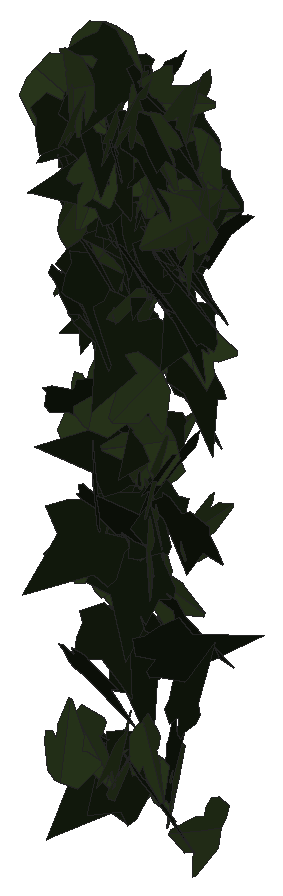
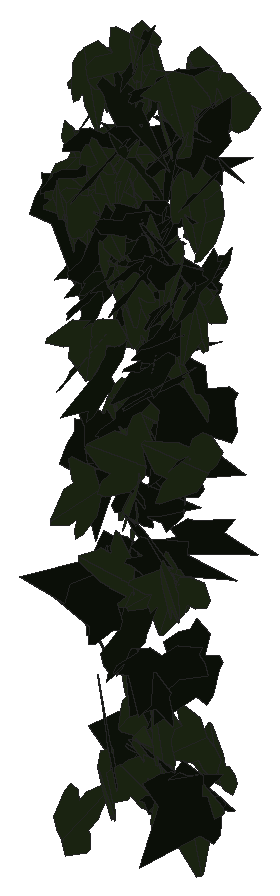
# SketchUp Ruby script. Lengths in inches.
U = 1.inch
M = Sketchup.active_model
def pt(a) = Geom::Point3d.new(a.map { |v| v * U })
def face(e, loops, mat)
  f = e.add_face(loops[0].map { |a| pt(a) })
  loops[1..].each { |l| e.add_face(l.map { |a| pt(a) }).erase! }
  f.material = f.back_material = mat if mat
  f
end
# faces: each face lists its corners as indices into pts; further lists are holes
def faces(e, pts, list, mat = nil) = list.each { |f| face(e, (f[0].is_a?(Array) ? f : [f]).map { |l| l.map { |i| pts[i] } }, mat) }
# xy, xz, yz: faces in a plane at the given z, y or x. An outline is a flat list of corners, or four numbers for a rectangle; further outlines are holes
def ring(l) = l.size == 4 ? [[l[0], l[1]], [l[2], l[1]], [l[2], l[3]], [l[0], l[3]]] : l.each_slice(2).to_a
def flat(e, list, mat, &to3) = list.each { |f| face(e, (f[0].is_a?(Array) ? f : [f]).map { |l| ring(l).map { |u, v| to3.(u, v) } }, mat) }
def xy(e, z, list, mat = nil) = flat(e, list, mat) { |x, y| [x, y, z] }
def xz(e, y, list, mat = nil) = flat(e, list, mat) { |x, z| [x, y, z] }
def yz(e, x, list, mat = nil) = flat(e, list, mat) { |y, z| [x, y, z] }
def lines(e, pts, list) = list.each { |a, b| e.add_line(pt(pts[a]), pt(pts[b])) }
# prism: a flat outline (further loops are holes) pulled along v
def prism(e, loops, v, mat = nil)
  f = face(e, loops, mat); d = Geom::Vector3d.new(v.map { |x| x * U })
  f.pushpull(f.normal.samedirection?(d) ? d.length : -d.length)
end
def box(e, o, s, mat = nil) = prism(e, [[o, [o[0] + s[0], o[1], o[2]], [o[0] + s[0], o[1] + s[1], o[2]], [o[0], o[1] + s[1], o[2]]]], [0, 0, s[2]], mat)
def at(x, y, z, deg = 0) = Geom::Transformation.translation(pt([x, y, z])) * Geom::Transformation.rotation(ORIGIN, Z_AXIS, deg.degrees)
def axes(o, x, y, z) = Geom::Transformation.new([*x, 0, *y, 0, *z, 0, *pt(o).to_a, 1])
def part(name) = M.definitions.add(name)
# library, detail: a bought-in or finely detailed component or shape, given as its bounding box
def library(name, o, s) = part(name).tap { |d| box(d.entities, o, s) }
def detail(e, o, s) = box(e.add_group.entities, o, s)
def put(e, d, t, mat = nil) = e.add_instance(d, t).tap { |i| i.material = mat if mat }
def group(e, t, mat = nil) = e.add_group.tap { |g| g.transformation = t; g.material = mat if mat }.entities
root = M.entities
M.materials.add("efeu1").color = [18, 25, 13]
M.materials.add("efeu2").color = [43, 57, 29]
c1 = part("ivyleaf_10")
p = [[0,0.5,-0.03],[-0.0625,2.02,-0.43],[-0.19,2.01,-0.46],[-0.54,1.05,-0.29],[-0.52,0.625,-0.18],[-0.83,0.76,-0.28],
  [-1.16,0.64,-0.33],[-1.15,0.33,-0.24],[-0.77,-0.39,0.02],[-0.3,-0.51,0.16],[0.04,-0.48,0.23],[-0.02,2.01,-0.4375],
  [-0.06,2.01,-0.43],[0.04,-0.49,0.23],[0.67,-0.49,0.14],[1.38,0.36,-0.2],[1.375,0.51,-0.24],[0.81,0.65,-0.19],
  [0.62,0.59,-0.15],[0.6,1.09,-0.28],[0.5,1.23,-0.31]]
faces(c1.entities,p,[[0,1,2,3,4,5,6,7,8,9,10],[11,12,0,13,14,15,16,17,18,19,20]],"efeu2")
c2 = part("ivyleaf_9")
p = [[1.54,2.16,1.25],[1.36,2.04,1.19],[-0.21,0.99,0.68],[-0.71,1.11,0.82],[-0.85,0.86,0.67],[-0.8,0.17,0.21],
  [-0.9,-0.01,0.1],[-0.67,-0.16,-0.02],[-0.08,-0.08,-0.05],[-0.03,-0.6,-0.4],[0.65,-0.88,-0.66],[0.83,-0.6,-0.49],
  [1.29,-0.42,-0.43],[1.8125,-0.07,-0.26],[1.21,0.44,0.15]]
faces(c2.entities,p,[[0,1,2,3,4,5,6,7,8,9,10,11,12,13,14]],"efeu1")
put(root,c1,axes([545.26,133.13,204.74],[-0.73909,0.23851,-0.3664],[0.3295,-0.16911,-0.77474],[-0.28734,-0.8074,0.05403]))
put(root,c1,axes([544.99,133.21,205.54],[0.29961,-0.81599,-0.04519],[-0.01203,0.04372,-0.86925],[0.81715,0.29983,0.00377]))
put(root,c2,axes([543.49,133.3125,192.88],[0.70059,0.05502,-0.37636],[0.37495,0.0327,0.70274],[0.06394,-0.79461,0.00286]))
put(root,c2,axes([544.64,133.57,199.95],[0.16686,-0.43211,0.71695],[0.45253,-0.56846,-0.44793],[0.70424,0.46767,0.11797]))
put(root,c2,axes([544.91,133.45,185.375],[0.48118,-0.55843,0.45126],[0.31159,-0.32699,-0.73689],[0.64683,0.57293,0.01927]))
put(root,c1,axes([545.18,133.15,197.3],[0.75679,-0.1709,-0.51183],[-0.48636,0.16585,-0.77451],[0.23373,0.89844,0.04562]))
put(root,c2,axes([543.22,133.73,191.91],[-0.63725,-0.47299,0.3462],[-0.25265,-0.2398,-0.79267],[0.52891,-0.68443,0.03847]))
put(root,c2,axes([542.52,133.125,199.37],[0.64655,-0.50733,-0.14909],[-0.09453,0.1208,-0.82105],[0.52027,0.65243,0.03609]))
put(root,c1,axes([543.21,132.95,205.28],[0.4039,-0.29481,-0.75471],[-0.61213,0.44146,-0.50005],[0.53084,0.73337,-0.00238]))
put(root,c2,axes([542.51,133.1,204.4375],[0.22259,-0.6267,-0.48664],[-0.07771,0.48577,-0.66114],[0.78964,0.22447,0.07211]))
put(root,c2,axes([544.32,133.73,198.39],[-0.53061,-0.67232,0.03547],[-0.01566,-0.03283,-0.85644],[0.67308,-0.53078,0.00804]))
put(root,c2,axes([545.4,133.03,205.05],[0.58579,-0.41864,-0.46192],[-0.30593,0.35923,-0.71354],[0.54317,0.65382,0.09628]))
put(root,c1,axes([543.05,133.1,204.71],[0.21401,-0.77882,-0.38187],[-0.10431,0.36736,-0.80768],[0.86111,0.23806,-0.00294]))
put(root,c1,axes([543.54,133.51,202.82],[0.44771,0.61092,-0.37702],[-0.20562,-0.31658,-0.75716],[-0.68781,0.4923,-0.01905]))
put(root,c2,axes([543.67,133.93,202.38],[-0.44901,-0.2473,0.7023],[-0.53972,-0.45686,-0.50594],[0.51292,-0.69722,0.08242]))
put(root,c2,axes([543.7,132.96,193.08],[0.0254,-0.26099,0.79603],[-0.07396,0.79259,0.26222],[-0.83446,-0.0782,0.00099]))
put(root,c1,axes([542.08,133.04,204.95],[0.42676,0.39564,0.752],[0.5705,0.49024,-0.58168],[-0.62973,0.71225,-0.01735]))
put(root,c1,axes([542.36,133.32,185.08],[0.83855,-0.13043,0.06033],[-0.05943,0.01043,0.84864],[-0.13085,-0.84066,0.00117]))
put(root,c1,axes([545.11,133.79,194.97],[0.46052,-0.62325,0.36788],[0.21487,-0.29863,-0.77492],[0.69109,0.50817,-0.00421]))
put(root,c1,axes([544.62,133.9,192.15],[-0.2474,0.36892,-0.73202],[0.31239,-0.6645,-0.44047],[-0.75788,-0.39433,0.0574]))
put(root,c1,axes([546.15,133.71,202.07],[-0.45461,-0.26856,0.6914],[-0.59262,-0.35615,-0.528],[0.44605,-0.7469,0.00316]))
put(root,c1,axes([543.24,133.42,195.62],[0.89242,-0.0937,-0.04669],[0.04644,-0.00485,0.89732],[-0.09383,-0.89363,0.00002]))
put(root,c1,axes([542.63,133.59,186.08],[0.49171,-0.02456,0.68501],[0.68531,0.03446,-0.49069],[-0.01369,0.84252,0.04004]))
put(root,c2,axes([542.83,133.29,188.33],[0.83916,-0.04245,-0.15527],[-0.15511,0.00708,-0.84024],[0.04303,0.85338,-0.00075]))
put(root,c2,axes([542.99,133.92,199.3],[0.14803,-0.85599,0.04688],[0.00548,-0.04663,-0.86869],[0.85725,0.14811,-0.00254]))
put(root,c1,axes([544.72,133.27,205.25],[0.13251,-0.7053,-0.48967],[-0.04739,0.4887,-0.71674],[0.85731,0.13603,0.03606]))
put(root,c2,axes([542.89,134.07,204.01],[0.07415,-0.85093,0.24891],[0.08796,-0.24149,-0.85175],[0.88221,0.0956,0.06401]))
put(root,c1,axes([543.62,133.83,204.17],[0.44375,-0.69965,0.2326],[0.12937,-0.19337,-0.82849],[0.72586,0.4622,0.00547]))
put(root,c2,axes([543.74,133.8,194.39],[-0.35876,0.03215,-0.71065],[-0.46719,-0.61085,0.20822],[-0.53645,0.51048,0.29391]))
put(root,c2,axes([546.09,133.41,193.57],[0.61284,0.18657,-0.5871],[-0.55834,-0.18167,-0.64056],[-0.26028,0.82901,-0.00825]))
put(root,c1,axes([544.5,133.85,186.39],[0.5136,-0.20518,0.64934],[0.63378,-0.15352,-0.5498],[0.24913,0.81355,0.06002]))
put(root,c1,axes([545.0625,133.74,195.23],[0.29192,0.05176,-0.75248],[-0.75328,-0.02097,-0.29367],[-0.0383,0.80684,0.04064]))
put(root,c1,axes([542.68,133.07,201.18],[0.15612,-0.25999,0.8628],[-0.41146,0.75847,0.303],[-0.8017,-0.43991,0.01251]))
put(root,c2,axes([542.8,133.26,196.11],[0.76405,0.57437,-0.04188],[-0.03362,-0.02498,-0.95586],[-0.57491,0.76479,0.00023]))
put(root,c2,axes([544.22,133.97,191.26],[-0.62604,-0.38377,-0.42316],[0.35019,0.23817,-0.7341],[0.45134,-0.71712,-0.01735]))
put(root,c2,axes([545.48,133.29,189.31],[0.38674,0.04129,0.82396],[0.7785,0.28292,-0.37958],[-0.27305,0.86513,0.08481]))
put(root,c2,axes([543.23,133.98,204.14],[-0.82081,0.04865,0.0752],[-0.07716,-0.03199,-0.82144],[-0.04548,-0.82362,0.03634]))
put(root,c2,axes([545.89,133.59,187.72],[-0.3688,0.59982,0.41627],[0.17633,-0.37938,0.70289],[0.7085,0.40664,0.04175]))
put(root,c2,axes([544.6,133.86,205.49],[0.56903,-0.60883,-0.02337],[-0.00629,0.0261,-0.83324],[0.60925,0.56891,0.01323]))
put(root,c2,axes([543.14,134.33,184.7],[-0.56529,-0.54835,0.28499],[-0.19588,-0.20733,-0.78746],[0.58612,-0.59815,0.01169]))
put(root,c2,axes([544.2,134.11,203.75],[0.38536,-0.74928,0.17655],[0.09013,-0.15217,-0.84251],[0.76451,0.39562,0.01033]))
put(root,c2,axes([543.06,133.83,203.65],[-0.36215,-0.3754,-0.68405],[0.4695,0.49752,-0.5216],[0.62324,-0.59293,-0.00456]))
put(root,c1,axes([543.8125,133.78,186.1],[0.2999,-0.88965,-0.21557],[-0.0663,0.20514,-0.93883],[0.91299,0.30713,0.00263]))
put(root,c2,axes([542.88,134.4,199.32],[-0.16641,-0.83006,0.24522],[-0.0451,-0.24106,-0.84657],[0.86435,-0.17239,0.00304]))
put(root,c1,axes([542.77,133.18,204.2],[0.03536,-0.15347,-0.87719],[-0.02897,0.87721,-0.15465],[0.89004,0.03465,0.02981]))
put(root,c2,axes([541.95,134.3,203.98],[-0.03631,-0.36872,0.77727],[0.45731,-0.66722,-0.29515],[0.72868,0.40036,0.22396]))
put(root,c2,axes([544.22,134,185.27],[-0.89094,0.21213,0.14268],[-0.13911,0.03176,-0.91585],[-0.21449,-0.90174,0.00131]))
put(root,c2,axes([543.39,134.47,205.5],[-0.43202,-0.68704,0.20937],[0.01096,-0.25061,-0.79974],[0.71815,-0.40948,0.13815]))
put(root,c1,axes([544,133.45,185.14],[0.37935,-0.47502,0.61192],[-0.20709,0.59437,0.58977],[-0.74646,-0.4063,0.14736]))
put(root,c1,axes([546.04,133.62,201.35],[0.51913,-0.39042,-0.56565],[-0.29599,0.51277,-0.62557],[0.62031,0.57142,0.17488]))
put(root,c1,axes([544.08,134.28,198.7],[0.05027,-0.79253,0.32776],[0.01841,-0.32725,-0.79412],[0.85743,0.05349,-0.00216]))
put(root,c2,axes([544.97,134,192.64],[-0.36227,0.10427,0.71846],[-0.69085,0.19728,-0.37698],[-0.22314,-0.78007,0.00069]))
put(root,c2,axes([545.38,134.04,194.77],[-0.38805,0.70584,-0.3151],[0.15047,-0.27685,-0.80548],[-0.7582,-0.4162,0.00142]))
put(root,c1,axes([544.87,133.5,205.08],[0.09087,0.04144,0.86809],[0.34663,0.79867,-0.07441],[-0.79696,0.3521,0.06661]))
put(root,c2,axes([542.4,134.1,202.4],[0.39181,-0.69102,-0.30617],[-0.12159,0.28275,-0.79375],[0.74597,0.40904,0.03143]))
put(root,c2,axes([544.45,134.73,195.43],[-0.22738,-0.66168,0.42526],[-0.14163,-0.40099,-0.69966],[0.7737,-0.26786,-0.0031]))
put(root,c2,axes([545.1,134.5625,198.66],[0.29652,-0.64631,0.47825],[0.24114,-0.41478,-0.71005],[0.767,0.38027,0.03835]))
put(root,c1,axes([544.37,134.24,193.26],[-0.42336,0.58806,-0.38068],[0.23513,-0.29971,-0.72447],[-0.65988,-0.48408,-0.01391]))
put(root,c2,axes([543.36,133.77,203.89],[0.34514,0.03695,-0.78352],[-0.76108,0.2229,-0.32475],[0.1898,0.82664,0.12259]))
put(root,c2,axes([545.3,134.87,198.83],[-0.16361,-0.68831,0.45102],[-0.0279,-0.45495,-0.70442],[0.82245,-0.15236,0.06582]))
put(root,c1,axes([542.78,134.24,199.53],[-0.65153,0.00173,0.47916],[-0.47436,-0.11656,-0.64458],[0.06768,-0.80031,0.09491]))
put(root,c1,axes([542.7,134.24,184.58],[-0.85532,-0.0793,0.43208],[-0.42979,-0.04455,-0.85897],[0.09086,-0.95722,0.00418]))
put(root,c1,axes([542.42,134.43,202.77],[0.02978,-0.835,-0.01775],[-0.0081,0.01748,-0.83549],[0.83515,0.02995,-0.00747]))
put(root,c2,axes([543.22,134.85,197.48],[-0.11185,0.03204,0.78495],[-0.01594,-0.7928,0.03009],[0.78544,-0.01152,0.11239]))
put(root,c1,axes([545.63,134.48,205.3],[0.03978,-0.84546,-0.01075],[0.01246,0.01134,-0.8463],[0.84544,0.03961,0.01298]))
put(root,c1,axes([544.48,134.47,190.57],[0.01134,-0.05015,0.84447],[0.84544,0.03013,-0.00957],[-0.02951,0.84401,0.05051]))
put(root,c2,axes([541.82,134.72,200.05],[0.39018,-0.6508,0.27175],[0.1751,-0.21145,-0.7578],[0.68318,0.42589,0.03902]))
put(root,c1,axes([542.29,134.18,199.47],[-0.11698,-0.72728,-0.411],[0.04774,0.40851,-0.73646],[0.83401,-0.12539,-0.01549]))
put(root,c2,axes([544.7,134.57,189.84],[0.57457,-0.35446,0.51902],[0.42482,-0.29923,-0.67465],[0.4632,0.71413,-0.02507]))
put(root,c1,axes([544.21,134.5,202.71],[-0.70565,-0.39815,0.0833],[-0.01467,-0.14177,-0.80193],[0.40651,-0.69626,0.11566]))
put(root,c2,axes([544.74,134.5625,200.58],[-0.60341,0.11226,0.59349],[-0.58622,0.09324,-0.61366],[-0.1455,-0.84121,0.01119]))
put(root,c2,axes([543.63,134.61,188.15],[-0.41231,-0.12852,-0.71929],[0.69162,0.19778,-0.43178],[0.2357,-0.80514,0.00875]))
put(root,c1,axes([544.08,134.59,185.01],[0.60264,0.19496,-0.51579],[-0.50873,-0.09817,-0.6315],[-0.21272,0.78713,0.04899]))
put(root,c2,axes([542.99,134.92,201.16],[0.18704,-0.76002,0.2687],[0.03922,-0.26693,-0.78232],[0.80517,0.18956,-0.02431]))
put(root,c1,axes([543.01,134.25,190.92],[0.44414,0.17752,0.63939],[0.5357,0.35813,-0.47155],[-0.39161,0.69124,0.08011]))
put(root,c2,axes([545.35,134.83,197.03],[0.26692,-0.78194,0.14398],[0.05403,-0.13369,-0.82621],[0.79325,0.27222,0.00783]))
put(root,c1,axes([545.93,134.32,202.47],[0.63157,-0.41535,-0.36935],[-0.18522,0.36983,-0.73262],[0.52405,0.63128,0.18618]))
put(root,c1,axes([542.5,133.95,194.29],[0.33461,0.38881,-0.75083],[0.50467,0.55604,0.51284],[0.6784,-0.60542,-0.01118]))
put(root,c2,axes([543.37,134.92,191.82],[-0.69139,-0.18242,0.44208],[-0.41893,-0.14383,-0.71453],[0.23068,-0.80794,0.02739]))
put(root,c2,axes([543.09,134.53,197.82],[-0.35852,-0.71787,0.36931],[0.22594,0.29872,0.79999],[-0.77504,0.41916,0.06238]))
put(root,c1,axes([545.66,135,202.08],[-0.24937,-0.52013,0.57878],[-0.0395,-0.59853,-0.55489],[0.77715,-0.19733,0.15751]))
put(root,c2,axes([544.54,134.79,185.04],[-0.06285,0.3839,0.76711],[0.12279,-0.75722,0.38901],[0.84898,0.13794,0.00052]))
put(root,c2,axes([544.53,134.34,203.32],[-0.50132,0.59775,0.24254],[-0.21572,0.13415,-0.77648],[-0.60794,-0.54051,0.07551]))
put(root,c1,axes([542.76,134.45,190.96],[0.63349,0.48756,0.24177],[0.1917,0.14733,-0.79939],[-0.50933,0.66186,-0.00016]))
put(root,c2,axes([544.52,134.54,200.06],[0.69505,-0.40928,0.03289],[0.03139,-0.01152,-0.80658],[0.4094,0.69573,0.006]))
put(root,c1,axes([544.55,134.96,200.51],[0.21843,-0.67264,0.43846],[0.14946,-0.41239,-0.70711],[0.7889,0.26437,0.01256]))
put(root,c2,axes([543.74,135.11,189.17],[0.69611,-0.36773,-0.47611],[0.41872,-0.22665,0.78726],[-0.43195,-0.81233,-0.00412]))
put(root,c2,axes([544.84,134.6,200.4],[0.66468,-0.45827,0.05261],[0.05435,-0.01384,-0.80712],[0.45807,0.66661,0.01942]))
put(root,c1,axes([542.8,134.57,205.73],[0.81786,0.08517,-0.1711],[-0.18267,0.12717,-0.80986],[-0.05622,0.82583,0.14236]))
put(root,c1,axes([544.23,134.41,203.18],[-0.34519,0.73963,0.09539],[-0.04707,0.08329,-0.81618],[-0.74427,-0.3483,0.00738]))
put(root,c1,axes([544.57,134.59,203.45],[-0.65232,-0.50228,-0.01359],[0.02977,-0.0164,-0.8227],[0.50158,-0.65226,0.03116]))
put(root,c1,axes([545.77,134.63,202.11],[-0.59518,-0.54617,0.01409],[-0.01007,-0.00987,-0.8078],[0.54626,-0.59527,0.00046]))
put(root,c2,axes([545.54,135.01,202.43],[-0.25025,-0.75614,-0.11815],[0.06084,0.10426,-0.79609],[0.7629,-0.25635,0.02473]))
put(root,c2,axes([544.51,134.67,205.01],[-0.601,0.58208,-0.13311],[0.0404,-0.14879,-0.83305],[-0.59574,-0.59731,0.07779]))
put(root,c2,axes([543.0625,135.29,196.84],[-0.35383,-0.60007,0.3717],[0.02258,-0.42519,-0.66494],[0.7055,-0.28734,0.2077]))
put(root,c2,axes([543,134.76,188.89],[-0.19994,-0.65934,-0.48241],[0.14031,0.46155,-0.68899],[0.80483,-0.24426,0.00027]))
put(root,c2,axes([543.52,135.25,199.83],[-0.0198,-0.7303,0.3051],[-0.00905,-0.30496,-0.73057],[0.79142,-0.02175,-0.00072]))
put(root,c2,axes([543.13,135.33,197.875],[-0.51569,-0.29361,0.53354],[-0.30766,-0.47775,-0.56028],[0.52556,-0.56777,0.19554]))
put(root,c2,axes([542.57,135.03,200.65],[-0.40549,-0.56768,-0.40989],[0.41348,0.18812,-0.66958],[0.56507,-0.54502,0.19582]))
put(root,c2,axes([544.66,134.99,203.78],[-0.37273,-0.6506,-0.34101],[0.16724,0.2972,-0.74981],[0.71527,-0.40852,-0.0024]))
put(root,c1,axes([544.32,134.27,193.96],[0.02351,-0.56616,0.73719],[-0.05312,0.7354,0.56648],[-0.92799,-0.05644,-0.01376]))
put(root,c1,axes([543.54,134.96,202.18],[0.67066,-0.44343,0.1329],[0.10443,-0.08299,-0.80392],[0.45098,0.67865,-0.01147]))
put(root,c2,axes([546.22,134.44,201.27],[-0.01981,0.81068,-0.01872],[0.00036,-0.01872,-0.81093],[-0.8109,-0.01981,0.0001]))
put(root,c1,axes([545.3,134.75,197.71],[0.53763,0.61433,0.05948],[0.03402,0.04926,-0.81634],[-0.61627,0.53866,0.00682]))
put(root,c2,axes([543.2,135.11,200.68],[0.05078,-0.79132,-0.07383],[0.11138,0.08034,-0.78445],[0.78692,0.03969,0.1158]))
put(root,c1,axes([545.44,135.47,183.34],[-0.06178,-0.25957,-0.81976],[-0.22394,-0.78866,0.26659],[-0.8302,0.23204,-0.01091]))
put(root,c2,axes([543.34,135.18,202.11],[-0.64328,-0.47837,-0.1466],[0.1193,0.08524,-0.80165],[0.4859,-0.65425,0.00275]))
put(root,c2,axes([542.11,134.36,184.91],[0.59422,0.51481,0.15954],[0.12371,0.10085,-0.7862],[-0.52458,0.60694,-0.00468]))
put(root,c2,axes([543.29,134.99,201.37],[-0.77798,0.21074,-0.10051],[0.10197,-0.00785,-0.80579],[-0.21003,-0.78441,-0.01894]))
put(root,c1,axes([542.53,135.125,191.58],[0.35921,-0.63716,0.27491],[0.18776,-0.20877,-0.72921],[0.66805,0.40128,0.05713]))
put(root,c1,axes([542.4,134.88,200.82],[-0.50228,0.58687,-0.24284],[0.13813,-0.20124,-0.77207],[-0.61992,-0.52034,0.02472]))
put(root,c1,axes([545.99,134.87,201.79],[0.16274,-0.81461,-0.12345],[-0.01821,0.12224,-0.83068],[0.8237,0.16364,0.00603]))
put(root,c2,axes([543.46,135.08,192.59],[-0.79308,0.12274,-0.25248],[0.24963,-0.03786,-0.80252],[-0.12844,-0.83144,-0.00072]))
put(root,c1,axes([545.44,134.99,203.3],[0.84462,-0.27428,-0.06915],[-0.06312,0.02949,-0.888],[0.27573,0.84693,0.00853]))
put(root,c2,axes([544.34,135.07,200.2],[0.43072,-0.65108,0.16732],[0.24832,-0.03056,-0.75817],[0.62469,0.46107,0.18601]))
put(root,c2,axes([542.88,134.8,197.92],[0.72534,-0.30458,-0.06604],[-0.05591,0.03739,-0.78659],[0.3066,0.72738,0.01279]))
put(root,c2,axes([544.55,134.98,196.7],[0.61849,-0.54837,-0.00221],[-0.00169,0.00142,-0.82659],[0.54838,0.6185,-0.00006]))
put(root,c1,axes([545.28,134.93,201.64],[0.64281,0.51287,0.03106],[0.027,0.01595,-0.82232],[-0.5131,0.64336,-0.00437]))
put(root,c2,axes([544.51,135.35,203.02],[0.14827,-0.78854,0.15368],[0.02799,-0.15111,-0.80236],[0.80289,0.15089,-0.00041]))
put(root,c2,axes([544.9375,134.71,199.79],[-0.39921,-0.5584,0.61929],[0.35701,0.50604,0.68642],[-0.75358,0.53556,-0.00288]))
put(root,c1,axes([544.49,135.26,185.08],[0.4445,-0.60257,0.35047],[0.2543,-0.24684,-0.74693],[0.64904,0.50939,0.05263]))
put(root,c1,axes([544.99,135.07,201.71],[-0.58113,-0.36356,0.42331],[-0.37011,-0.20626,-0.68524],[0.41759,-0.68874,-0.01823]))
put(root,c1,axes([545.73,134.33,192.53],[0.1789,-0.03798,0.82931],[-0.23732,0.8106,0.08832],[-0.79553,-0.25036,0.16015]))
put(root,c1,axes([544.07,135.07,199.89],[0.79316,-0.07394,-0.01763],[-0.01783,-0.00127,-0.7966],[0.07389,0.79336,-0.00292]))
put(root,c2,axes([543.68,135.4375,201.8],[-0.51919,-0.62151,-0.03766],[0.11773,-0.04984,-0.80056],[0.61142,-0.51816,0.12218]))
